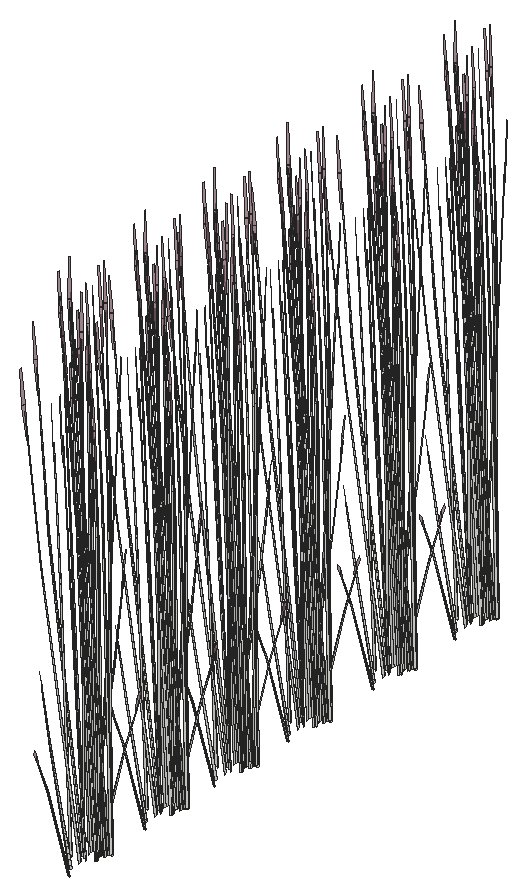
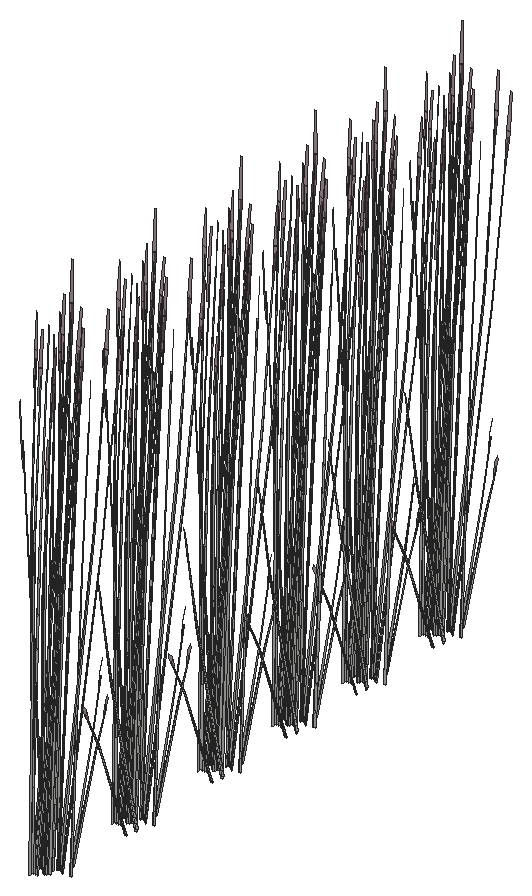
# SketchUp Ruby script. Lengths in inches.
U = 1.inch
M = Sketchup.active_model
def pt(a) = Geom::Point3d.new(a.map { |v| v * U })
def face(e, loops, mat)
  f = e.add_face(loops[0].map { |a| pt(a) })
  loops[1..].each { |l| e.add_face(l.map { |a| pt(a) }).erase! }
  f.material = f.back_material = mat if mat
  f
end
# faces: each face lists its corners as indices into pts; further lists are holes
def faces(e, pts, list, mat = nil) = list.each { |f| face(e, (f[0].is_a?(Array) ? f : [f]).map { |l| l.map { |i| pts[i] } }, mat) }
# xy, xz, yz: faces in a plane at the given z, y or x. An outline is a flat list of corners, or four numbers for a rectangle; further outlines are holes
def ring(l) = l.size == 4 ? [[l[0], l[1]], [l[2], l[1]], [l[2], l[3]], [l[0], l[3]]] : l.each_slice(2).to_a
def flat(e, list, mat, &to3) = list.each { |f| face(e, (f[0].is_a?(Array) ? f : [f]).map { |l| ring(l).map { |u, v| to3.(u, v) } }, mat) }
def xy(e, z, list, mat = nil) = flat(e, list, mat) { |x, y| [x, y, z] }
def xz(e, y, list, mat = nil) = flat(e, list, mat) { |x, z| [x, y, z] }
def yz(e, x, list, mat = nil) = flat(e, list, mat) { |y, z| [x, y, z] }
def lines(e, pts, list) = list.each { |a, b| e.add_line(pt(pts[a]), pt(pts[b])) }
# prism: a flat outline (further loops are holes) pulled along v
def prism(e, loops, v, mat = nil)
  f = face(e, loops, mat); d = Geom::Vector3d.new(v.map { |x| x * U })
  f.pushpull(f.normal.samedirection?(d) ? d.length : -d.length)
end
def box(e, o, s, mat = nil) = prism(e, [[o, [o[0] + s[0], o[1], o[2]], [o[0] + s[0], o[1] + s[1], o[2]], [o[0], o[1] + s[1], o[2]]]], [0, 0, s[2]], mat)
def at(x, y, z, deg = 0) = Geom::Transformation.translation(pt([x, y, z])) * Geom::Transformation.rotation(ORIGIN, Z_AXIS, deg.degrees)
def axes(o, x, y, z) = Geom::Transformation.new([*x, 0, *y, 0, *z, 0, *pt(o).to_a, 1])
def part(name) = M.definitions.add(name)
# library, detail: a bought-in or finely detailed component or shape, given as its bounding box
def library(name, o, s) = part(name).tap { |d| box(d.entities, o, s) }
def detail(e, o, s) = box(e.add_group.entities, o, s)
def put(e, d, t, mat = nil) = e.add_instance(d, t).tap { |i| i.material = mat if mat }
def group(e, t, mat = nil) = e.add_group.tap { |g| g.transformation = t; g.material = mat if mat }.entities
root = M.entities
M.materials.add("LightPink_Translucent").color = [144, 107, 117]
M.materials["LightPink_Translucent"].alpha = 0.75
c1 = part("blade")
p = [[2.15,0.21,22],[0,0.17,0],[0.09,0.45,0],[2.18,0.31,22],[2.29,0.31,22],[0.38,0.45,0],
  [2.48,0.24,33],[2.49,0.24,33],[2.48,0.22,33]]
faces(c1.entities,p,[[0,1,2,3],[4,5,2,3],[6,3,4,7],[8,0,3,6]])
c2 = part("seeds")
p = [[0.3,-0.1,1.38],[-0.01,-0.03,1.59],[-0.01,-0.03,0.03],[0.14,-0.07,-0.07],[0.29,-0.03,3],[0.15,0.01,3.11]]
faces(c2.entities,p,[[0,1,2,3],[1,0,4,5]],"LightPink_Translucent")
c3 = part("blade with seeds")
put(c3.entities,c1,at(0,0,0))
put(c3.entities,c2,axes([2.4,0.25,30.99],[1.5799,-0.05474,1.17369],[-0.12525,1.92788,0.29478],[-0.07173,-0.02425,1.56792]))
put(root,c3,axes([333.7,274.53,49.32],[-0.08469,0.01408,1.55816],[-0.46834,-0.15847,-0.23804],[0.00786,-0.13218,0.26541]))
put(root,c3,axes([333,276.42,49.85],[-0.20736,-0.4007,-0.61707],[0.59731,-0.14431,-0.16195],[-0.02292,-0.13569,1.36206]))
put(root,c3,axes([333.61,274.8,49.88],[-0.34892,0.22417,-0.0344],[-0.3197,-0.24551,-0.15595],[-0.02251,-0.06957,0.51438]))
put(root,c3,axes([333.32,276.53,49.95],[0.24498,-0.3521,-0.39531],[0.50902,0.16945,0.19025],[0,-0.08116,1.26923]))
put(root,c3,axes([332.02,276.375,49.79],[0.35245,-0.2438,-0.27372],[0.35245,0.2438,0.27372],[0,-0.07853,1.22797]))
put(root,c3,axes([333.25,276.82,50.36],[-0.56863,-0.18645,-0.25709],[0.2738,-0.39352,-0.44182],[-0.01787,-0.09662,1.41118]))
put(root,c3,axes([333.42,276.58,50.09],[0.21952,0.43694,0.40429],[-0.62724,0.15194,0.15865],[0.00767,-0.08029,1.40366]))
put(root,c3,axes([333.31,276.93,50.4],[-0.24498,0.3521,0.39531],[-0.50902,-0.16945,-0.19025],[0,-0.08116,1.26923]))
put(root,c3,axes([334.36,276.97,50.03],[-0.46965,-0.33633,-0.05417],[0.46994,-0.33653,0],[-0.0164,-0.01174,1.55135]))
put(root,c3,axes([333.47,277.01,50.09],[0.63817,0.08233,0.40429],[-0.12987,0.46497,0.15865],[-0.09326,-0.0449,1.40366]))
put(root,c3,axes([333.13,277.75,50.1875],[0.54257,-0.10371,0.15589],[0.13397,0.38597,0.31002],[-0.04839,-0.05624,1.41735]))
put(root,c3,axes([333.94,277.66,49.95],[-0.16474,-0.33688,0],[0.47043,-0.11798,0],[0,0,1.36402]))
put(root,c3,axes([334.74,277.77,50.1875],[0.14586,-0.38834,0.15589],[0.53375,0.1099,0.31002],[-0.0922,0.00189,1.41735]))
put(root,c3,axes([333.83,277.82,49.94],[-0.50902,-0.17543,0],[0.24498,-0.36452,0],[0,0,1.43768]))
put(root,c3,axes([334.49,277.09,50.4],[0.54829,-0.02412,0.39531],[0.04958,0.40041,-0.19025],[-0.09816,0.04058,1.26923]))
put(root,c3,axes([334.61,278.21,49.9375],[-0.31175,-0.39292,-0.04544],[0.52815,-0.21836,0.456],[-0.13015,0.03741,1.44584]))
put(root,c3,axes([334.5,277.26,50.3125],[0.37303,0.23477,0.12794],[-0.31115,0.26487,-0.36534],[-0.08661,0.03581,1.11991]))
put(root,c3,axes([334.89,277.98,50.19],[0.47255,-0.19538,0.43871],[0.28245,0.35034,0],[-0.10763,0.0445,1.3917]))
put(root,c3,axes([334.46,278.16,49.79],[-0.47106,-0.09668,-0.27372],[0.11861,-0.34048,0.27372],[-0.09497,0.03926,1.22797]))
put(root,c3,axes([334.38,277.17,50.36],[0.05884,0.44587,-0.25709],[-0.6128,0.02696,-0.44182],[-0.10791,0.05939,1.41118]))
put(root,c3,axes([334.61,277,49.95],[-0.24498,0.3521,-0.39531],[-0.50902,-0.16945,0.19025],[0,0.08116,1.26923]))
put(root,c3,axes([334.62,278.01,50.06],[0.63212,0.12701,0.27176],[-0.15814,0.45398,-0.32244],[-0.10462,0.05682,1.45692]))
put(root,c3,axes([335,278.25,50.1],[0.31568,0.39156,0],[-0.52815,0.21836,-0.456],[-0.12029,0.04973,1.44655]))
put(root,c3,axes([333.34,278.375,49.32],[0.08172,-0.02126,1.55816],[0.49154,0.11703,-0.23804],[0.01437,0.1319,0.26541]))
put(root,c3,axes([332.21,278.43,50.49],[0.45869,-0.0692,0.0575],[0.10545,0.27878,-0.76259],[-0.02908,0.14112,0.68355]))
put(root,c3,axes([333.7,284.33,49.32],[-0.08469,0.01408,1.55816],[-0.46834,-0.15847,-0.23804],[0.00786,-0.13218,0.26541]))
put(root,c3,axes([333,286.23,49.85],[-0.20736,-0.4007,-0.61707],[0.59731,-0.14431,-0.16195],[-0.02292,-0.13569,1.36206]))
put(root,c3,axes([333.61,284.6,49.88],[-0.34892,0.22417,-0.0344],[-0.3197,-0.24551,-0.15595],[-0.02251,-0.06957,0.51438]))
put(root,c3,axes([333.32,286.33,49.95],[0.24498,-0.3521,-0.39531],[0.50902,0.16945,0.19025],[0,-0.08116,1.26923]))
put(root,c3,axes([332.02,286.18,49.79],[0.35245,-0.2438,-0.27372],[0.35245,0.2438,0.27372],[0,-0.07853,1.22797]))
put(root,c3,axes([333.25,286.62,50.36],[-0.56863,-0.18645,-0.25709],[0.2738,-0.39352,-0.44182],[-0.01787,-0.09662,1.41118]))
put(root,c3,axes([333.42,286.38,50.09],[0.21952,0.43694,0.40429],[-0.62724,0.15194,0.15865],[0.00767,-0.08029,1.40366]))
put(root,c3,axes([333.31,286.73,50.4],[-0.24498,0.3521,0.39531],[-0.50902,-0.16945,-0.19025],[0,-0.08116,1.26923]))
put(root,c3,axes([334.36,286.77,50.03],[-0.46965,-0.33633,-0.05417],[0.46994,-0.33653,0],[-0.0164,-0.01174,1.55135]))
put(root,c3,axes([333.47,286.8125,50.09],[0.63817,0.08233,0.40429],[-0.12987,0.46497,0.15865],[-0.09326,-0.0449,1.40366]))
put(root,c3,axes([333.13,287.56,50.1875],[0.54257,-0.10371,0.15589],[0.13397,0.38597,0.31002],[-0.04839,-0.05624,1.41735]))
put(root,c3,axes([333.94,287.46,49.95],[-0.16474,-0.33688,0],[0.47043,-0.11798,0],[0,0,1.36402]))
put(root,c3,axes([334.74,287.58,50.1875],[0.14586,-0.38834,0.15589],[0.53375,0.1099,0.31002],[-0.0922,0.00189,1.41735]))
put(root,c3,axes([333.83,287.62,49.94],[-0.50902,-0.17543,0],[0.24498,-0.36452,0],[0,0,1.43768]))
put(root,c3,axes([334.49,286.89,50.4],[0.54829,-0.02412,0.39531],[0.04958,0.40041,-0.19025],[-0.09816,0.04058,1.26923]))
put(root,c3,axes([334.61,288.01,49.9375],[-0.31175,-0.39292,-0.04544],[0.52815,-0.21836,0.456],[-0.13015,0.03741,1.44584]))
put(root,c3,axes([334.5,287.0625,50.3125],[0.37303,0.23477,0.12794],[-0.31115,0.26487,-0.36534],[-0.08661,0.03581,1.11991]))
put(root,c3,axes([334.89,287.79,50.19],[0.47255,-0.19538,0.43871],[0.28245,0.35034,0],[-0.10763,0.0445,1.3917]))
put(root,c3,axes([334.46,287.96,49.79],[-0.47106,-0.09668,-0.27372],[0.11861,-0.34048,0.27372],[-0.09497,0.03926,1.22797]))
put(root,c3,axes([334.38,286.97,50.36],[0.05884,0.44587,-0.25709],[-0.6128,0.02696,-0.44182],[-0.10791,0.05939,1.41118]))
put(root,c3,axes([334.61,286.8,49.95],[-0.24498,0.3521,-0.39531],[-0.50902,-0.16945,0.19025],[0,0.08116,1.26923]))
put(root,c3,axes([334.62,287.81,50.06],[0.63212,0.12701,0.27176],[-0.15814,0.45398,-0.32244],[-0.10462,0.05682,1.45692]))
put(root,c3,axes([335,288.06,50.1],[0.31568,0.39156,0],[-0.52815,0.21836,-0.456],[-0.12029,0.04973,1.44655]))
put(root,c3,axes([333.34,288.18,49.32],[0.08172,-0.02126,1.55816],[0.49154,0.11703,-0.23804],[0.01437,0.1319,0.26541]))
put(root,c3,axes([332.21,288.23,50.49],[0.45869,-0.0692,0.0575],[0.10545,0.27878,-0.76259],[-0.02908,0.14112,0.68355]))
put(root,c3,axes([333.7,293.3,49.32],[-0.08469,0.01408,1.55816],[-0.46834,-0.15847,-0.23804],[0.00786,-0.13218,0.26541]))
put(root,c3,axes([333,295.2,49.85],[-0.20736,-0.4007,-0.61707],[0.59731,-0.14431,-0.16195],[-0.02292,-0.13569,1.36206]))
put(root,c3,axes([333.61,293.58,49.88],[-0.34892,0.22417,-0.0344],[-0.3197,-0.24551,-0.15595],[-0.02251,-0.06957,0.51438]))
put(root,c3,axes([333.32,295.31,49.95],[0.24498,-0.3521,-0.39531],[0.50902,0.16945,0.19025],[0,-0.08116,1.26923]))
put(root,c3,axes([332.02,295.16,49.79],[0.35245,-0.2438,-0.27372],[0.35245,0.2438,0.27372],[0,-0.07853,1.22797]))
put(root,c3,axes([333.25,295.6,50.36],[-0.56863,-0.18645,-0.25709],[0.2738,-0.39352,-0.44182],[-0.01787,-0.09662,1.41118]))
put(root,c3,axes([333.42,295.36,50.09],[0.21952,0.43694,0.40429],[-0.62724,0.15194,0.15865],[0.00767,-0.08029,1.40366]))
put(root,c3,axes([333.31,295.71,50.4],[-0.24498,0.3521,0.39531],[-0.50902,-0.16945,-0.19025],[0,-0.08116,1.26923]))
put(root,c3,axes([334.36,295.75,50.03],[-0.46965,-0.33633,-0.05417],[0.46994,-0.33653,0],[-0.0164,-0.01174,1.55135]))
put(root,c3,axes([333.47,295.79,50.09],[0.63817,0.08233,0.40429],[-0.12987,0.46497,0.15865],[-0.09326,-0.0449,1.40366]))
put(root,c3,axes([333.13,296.53,50.1875],[0.54257,-0.10371,0.15589],[0.13397,0.38597,0.31002],[-0.04839,-0.05624,1.41735]))
put(root,c3,axes([333.94,296.44,49.95],[-0.16474,-0.33688,0],[0.47043,-0.11798,0],[0,0,1.36402]))
put(root,c3,axes([334.74,296.55,50.1875],[0.14586,-0.38834,0.15589],[0.53375,0.1099,0.31002],[-0.0922,0.00189,1.41735]))
put(root,c3,axes([333.83,296.59,49.94],[-0.50902,-0.17543,0],[0.24498,-0.36452,0],[0,0,1.43768]))
put(root,c3,axes([334.49,295.87,50.4],[0.54829,-0.02412,0.39531],[0.04958,0.40041,-0.19025],[-0.09816,0.04058,1.26923]))
put(root,c3,axes([334.61,296.99,49.9375],[-0.31175,-0.39292,-0.04544],[0.52815,-0.21836,0.456],[-0.13015,0.03741,1.44584]))
put(root,c3,axes([334.5,296.04,50.3125],[0.37303,0.23477,0.12794],[-0.31115,0.26487,-0.36534],[-0.08661,0.03581,1.11991]))
put(root,c3,axes([334.89,296.76,50.19],[0.47255,-0.19538,0.43871],[0.28245,0.35034,0],[-0.10763,0.0445,1.3917]))
put(root,c3,axes([334.46,296.9375,49.79],[-0.47106,-0.09668,-0.27372],[0.11861,-0.34048,0.27372],[-0.09497,0.03926,1.22797]))
put(root,c3,axes([334.38,295.95,50.36],[0.05884,0.44587,-0.25709],[-0.6128,0.02696,-0.44182],[-0.10791,0.05939,1.41118]))
put(root,c3,axes([334.61,295.78,49.95],[-0.24498,0.3521,-0.39531],[-0.50902,-0.16945,0.19025],[0,0.08116,1.26923]))
put(root,c3,axes([334.62,296.79,50.06],[0.63212,0.12701,0.27176],[-0.15814,0.45398,-0.32244],[-0.10462,0.05682,1.45692]))
put(root,c3,axes([335,297.03,50.1],[0.31568,0.39156,0],[-0.52815,0.21836,-0.456],[-0.12029,0.04973,1.44655]))
put(root,c3,axes([333.34,297.15,49.32],[0.08172,-0.02126,1.55816],[0.49154,0.11703,-0.23804],[0.01437,0.1319,0.26541]))
put(root,c3,axes([332.21,297.21,50.49],[0.45869,-0.0692,0.0575],[0.10545,0.27878,-0.76259],[-0.02908,0.14112,0.68355]))
put(root,c3,axes([333.7,302.79,49.32],[-0.08469,0.01408,1.55816],[-0.46834,-0.15847,-0.23804],[0.00786,-0.13218,0.26541]))
put(root,c3,axes([333,304.6875,49.85],[-0.20736,-0.4007,-0.61707],[0.59731,-0.14431,-0.16195],[-0.02292,-0.13569,1.36206]))
put(root,c3,axes([333.61,303.0625,49.88],[-0.34892,0.22417,-0.0344],[-0.3197,-0.24551,-0.15595],[-0.02251,-0.06957,0.51438]))
put(root,c3,axes([333.32,304.79,49.95],[0.24498,-0.3521,-0.39531],[0.50902,0.16945,0.19025],[0,-0.08116,1.26923]))
put(root,c3,axes([332.02,304.64,49.79],[0.35245,-0.2438,-0.27372],[0.35245,0.2438,0.27372],[0,-0.07853,1.22797]))
put(root,c3,axes([333.25,305.08,50.36],[-0.56863,-0.18645,-0.25709],[0.2738,-0.39352,-0.44182],[-0.01787,-0.09662,1.41118]))
put(root,c3,axes([333.42,304.85,50.09],[0.21952,0.43694,0.40429],[-0.62724,0.15194,0.15865],[0.00767,-0.08029,1.40366]))
put(root,c3,axes([333.31,305.19,50.4],[-0.24498,0.3521,0.39531],[-0.50902,-0.16945,-0.19025],[0,-0.08116,1.26923]))
put(root,c3,axes([334.36,305.23,50.03],[-0.46965,-0.33633,-0.05417],[0.46994,-0.33653,0],[-0.0164,-0.01174,1.55135]))
put(root,c3,axes([333.47,305.27,50.09],[0.63817,0.08233,0.40429],[-0.12987,0.46497,0.15865],[-0.09326,-0.0449,1.40366]))
put(root,c3,axes([333.13,306.02,50.1875],[0.54257,-0.10371,0.15589],[0.13397,0.38597,0.31002],[-0.04839,-0.05624,1.41735]))
put(root,c3,axes([333.94,305.93,49.95],[-0.16474,-0.33688,0],[0.47043,-0.11798,0],[0,0,1.36402]))
put(root,c3,axes([334.74,306.04,50.1875],[0.14586,-0.38834,0.15589],[0.53375,0.1099,0.31002],[-0.0922,0.00189,1.41735]))
put(root,c3,axes([333.83,306.08,49.94],[-0.50902,-0.17543,0],[0.24498,-0.36452,0],[0,0,1.43768]))
put(root,c3,axes([334.49,305.35,50.4],[0.54829,-0.02412,0.39531],[0.04958,0.40041,-0.19025],[-0.09816,0.04058,1.26923]))
put(root,c3,axes([334.61,306.47,49.9375],[-0.31175,-0.39292,-0.04544],[0.52815,-0.21836,0.456],[-0.13015,0.03741,1.44584]))
put(root,c3,axes([334.5,305.52,50.3125],[0.37303,0.23477,0.12794],[-0.31115,0.26487,-0.36534],[-0.08661,0.03581,1.11991]))
put(root,c3,axes([334.89,306.25,50.19],[0.47255,-0.19538,0.43871],[0.28245,0.35034,0],[-0.10763,0.0445,1.3917]))
put(root,c3,axes([334.46,306.42,49.79],[-0.47106,-0.09668,-0.27372],[0.11861,-0.34048,0.27372],[-0.09497,0.03926,1.22797]))
put(root,c3,axes([334.38,305.4375,50.36],[0.05884,0.44587,-0.25709],[-0.6128,0.02696,-0.44182],[-0.10791,0.05939,1.41118]))
put(root,c3,axes([334.61,305.26,49.95],[-0.24498,0.3521,-0.39531],[-0.50902,-0.16945,0.19025],[0,0.08116,1.26923]))
put(root,c3,axes([334.62,306.27,50.06],[0.63212,0.12701,0.27176],[-0.15814,0.45398,-0.32244],[-0.10462,0.05682,1.45692]))
put(root,c3,axes([335,306.52,50.1],[0.31568,0.39156,0],[-0.52815,0.21836,-0.456],[-0.12029,0.04973,1.44655]))
put(root,c3,axes([333.34,306.64,49.32],[0.08172,-0.02126,1.55816],[0.49154,0.11703,-0.23804],[0.01437,0.1319,0.26541]))
put(root,c3,axes([332.21,306.69,50.49],[0.45869,-0.0692,0.0575],[0.10545,0.27878,-0.76259],[-0.02908,0.14112,0.68355]))
put(root,c3,axes([333.7,313.78,49.32],[-0.08469,0.01408,1.55816],[-0.46834,-0.15847,-0.23804],[0.00786,-0.13218,0.26541]))
put(root,c3,axes([333,315.68,49.85],[-0.20736,-0.4007,-0.61707],[0.59731,-0.14431,-0.16195],[-0.02292,-0.13569,1.36206]))
put(root,c3,axes([333.61,314.05,49.88],[-0.34892,0.22417,-0.0344],[-0.3197,-0.24551,-0.15595],[-0.02251,-0.06957,0.51438]))
put(root,c3,axes([333.32,315.78,49.95],[0.24498,-0.3521,-0.39531],[0.50902,0.16945,0.19025],[0,-0.08116,1.26923]))
put(root,c3,axes([332.02,315.63,49.79],[0.35245,-0.2438,-0.27372],[0.35245,0.2438,0.27372],[0,-0.07853,1.22797]))
put(root,c3,axes([333.25,316.07,50.36],[-0.56863,-0.18645,-0.25709],[0.2738,-0.39352,-0.44182],[-0.01787,-0.09662,1.41118]))
put(root,c3,axes([333.42,315.84,50.09],[0.21952,0.43694,0.40429],[-0.62724,0.15194,0.15865],[0.00767,-0.08029,1.40366]))
put(root,c3,axes([333.31,316.18,50.4],[-0.24498,0.3521,0.39531],[-0.50902,-0.16945,-0.19025],[0,-0.08116,1.26923]))
put(root,c3,axes([334.36,316.22,50.03],[-0.46965,-0.33633,-0.05417],[0.46994,-0.33653,0],[-0.0164,-0.01174,1.55135]))
put(root,c3,axes([333.47,316.26,50.09],[0.63817,0.08233,0.40429],[-0.12987,0.46497,0.15865],[-0.09326,-0.0449,1.40366]))
put(root,c3,axes([333.13,317.01,50.1875],[0.54257,-0.10371,0.15589],[0.13397,0.38597,0.31002],[-0.04839,-0.05624,1.41735]))
put(root,c3,axes([333.94,316.92,49.95],[-0.16474,-0.33688,0],[0.47043,-0.11798,0],[0,0,1.36402]))
put(root,c3,axes([334.74,317.03,50.1875],[0.14586,-0.38834,0.15589],[0.53375,0.1099,0.31002],[-0.0922,0.00189,1.41735]))
put(root,c3,axes([333.83,317.07,49.94],[-0.50902,-0.17543,0],[0.24498,-0.36452,0],[0,0,1.43768]))
put(root,c3,axes([334.49,316.34,50.4],[0.54829,-0.02412,0.39531],[0.04958,0.40041,-0.19025],[-0.09816,0.04058,1.26923]))
put(root,c3,axes([334.61,317.46,49.9375],[-0.31175,-0.39292,-0.04544],[0.52815,-0.21836,0.456],[-0.13015,0.03741,1.44584]))
put(root,c3,axes([334.5,316.51,50.3125],[0.37303,0.23477,0.12794],[-0.31115,0.26487,-0.36534],[-0.08661,0.03581,1.11991]))
put(root,c3,axes([334.89,317.24,50.19],[0.47255,-0.19538,0.43871],[0.28245,0.35034,0],[-0.10763,0.0445,1.3917]))
put(root,c3,axes([334.46,317.41,49.79],[-0.47106,-0.09668,-0.27372],[0.11861,-0.34048,0.27372],[-0.09497,0.03926,1.22797]))
put(root,c3,axes([334.38,316.43,50.36],[0.05884,0.44587,-0.25709],[-0.6128,0.02696,-0.44182],[-0.10791,0.05939,1.41118]))
put(root,c3,axes([334.61,316.25,49.95],[-0.24498,0.3521,-0.39531],[-0.50902,-0.16945,0.19025],[0,0.08116,1.26923]))
put(root,c3,axes([334.62,317.26,50.06],[0.63212,0.12701,0.27176],[-0.15814,0.45398,-0.32244],[-0.10462,0.05682,1.45692]))
put(root,c3,axes([335,317.51,50.1],[0.31568,0.39156,0],[-0.52815,0.21836,-0.456],[-0.12029,0.04973,1.44655]))
put(root,c3,axes([333.34,317.625,49.32],[0.08172,-0.02126,1.55816],[0.49154,0.11703,-0.23804],[0.01437,0.1319,0.26541]))
put(root,c3,axes([332.21,317.68,50.49],[0.45869,-0.0692,0.0575],[0.10545,0.27878,-0.76259],[-0.02908,0.14112,0.68355]))
put(root,c3,axes([333.7,324.375,49.32],[-0.08469,0.01408,1.55816],[-0.46834,-0.15847,-0.23804],[0.00786,-0.13218,0.26541]))
put(root,c3,axes([333,326.27,49.85],[-0.20736,-0.4007,-0.61707],[0.59731,-0.14431,-0.16195],[-0.02292,-0.13569,1.36206]))
put(root,c3,axes([333.61,324.65,49.88],[-0.34892,0.22417,-0.0344],[-0.3197,-0.24551,-0.15595],[-0.02251,-0.06957,0.51438]))
put(root,c3,axes([333.32,326.38,49.95],[0.24498,-0.3521,-0.39531],[0.50902,0.16945,0.19025],[0,-0.08116,1.26923]))
put(root,c3,axes([332.02,326.23,49.79],[0.35245,-0.2438,-0.27372],[0.35245,0.2438,0.27372],[0,-0.07853,1.22797]))
put(root,c3,axes([333.25,326.67,50.36],[-0.56863,-0.18645,-0.25709],[0.2738,-0.39352,-0.44182],[-0.01787,-0.09662,1.41118]))
put(root,c3,axes([333.42,326.43,50.09],[0.21952,0.43694,0.40429],[-0.62724,0.15194,0.15865],[0.00767,-0.08029,1.40366]))
put(root,c3,axes([333.31,326.78,50.4],[-0.24498,0.3521,0.39531],[-0.50902,-0.16945,-0.19025],[0,-0.08116,1.26923]))
put(root,c3,axes([334.36,326.82,50.03],[-0.46965,-0.33633,-0.05417],[0.46994,-0.33653,0],[-0.0164,-0.01174,1.55135]))
put(root,c3,axes([333.47,326.86,50.09],[0.63817,0.08233,0.40429],[-0.12987,0.46497,0.15865],[-0.09326,-0.0449,1.40366]))
put(root,c3,axes([333.13,327.6,50.1875],[0.54257,-0.10371,0.15589],[0.13397,0.38597,0.31002],[-0.04839,-0.05624,1.41735]))
put(root,c3,axes([333.94,327.51,49.95],[-0.16474,-0.33688,0],[0.47043,-0.11798,0],[0,0,1.36402]))
put(root,c3,axes([334.74,327.625,50.1875],[0.14586,-0.38834,0.15589],[0.53375,0.1099,0.31002],[-0.0922,0.00189,1.41735]))
put(root,c3,axes([333.83,327.67,49.94],[-0.50902,-0.17543,0],[0.24498,-0.36452,0],[0,0,1.43768]))
put(root,c3,axes([334.49,326.9375,50.4],[0.54829,-0.02412,0.39531],[0.04958,0.40041,-0.19025],[-0.09816,0.04058,1.26923]))
put(root,c3,axes([334.61,328.06,49.9375],[-0.31175,-0.39292,-0.04544],[0.52815,-0.21836,0.456],[-0.13015,0.03741,1.44584]))
put(root,c3,axes([334.5,327.11,50.3125],[0.37303,0.23477,0.12794],[-0.31115,0.26487,-0.36534],[-0.08661,0.03581,1.11991]))
put(root,c3,axes([334.89,327.83,50.19],[0.47255,-0.19538,0.43871],[0.28245,0.35034,0],[-0.10763,0.0445,1.3917]))
put(root,c3,axes([334.46,328.01,49.79],[-0.47106,-0.09668,-0.27372],[0.11861,-0.34048,0.27372],[-0.09497,0.03926,1.22797]))
put(root,c3,axes([334.38,327.02,50.36],[0.05884,0.44587,-0.25709],[-0.6128,0.02696,-0.44182],[-0.10791,0.05939,1.41118]))
put(root,c3,axes([334.61,326.85,49.95],[-0.24498,0.3521,-0.39531],[-0.50902,-0.16945,0.19025],[0,0.08116,1.26923]))
put(root,c3,axes([334.62,327.86,50.06],[0.63212,0.12701,0.27176],[-0.15814,0.45398,-0.32244],[-0.10462,0.05682,1.45692]))
put(root,c3,axes([335,328.1,50.1],[0.31568,0.39156,0],[-0.52815,0.21836,-0.456],[-0.12029,0.04973,1.44655]))
